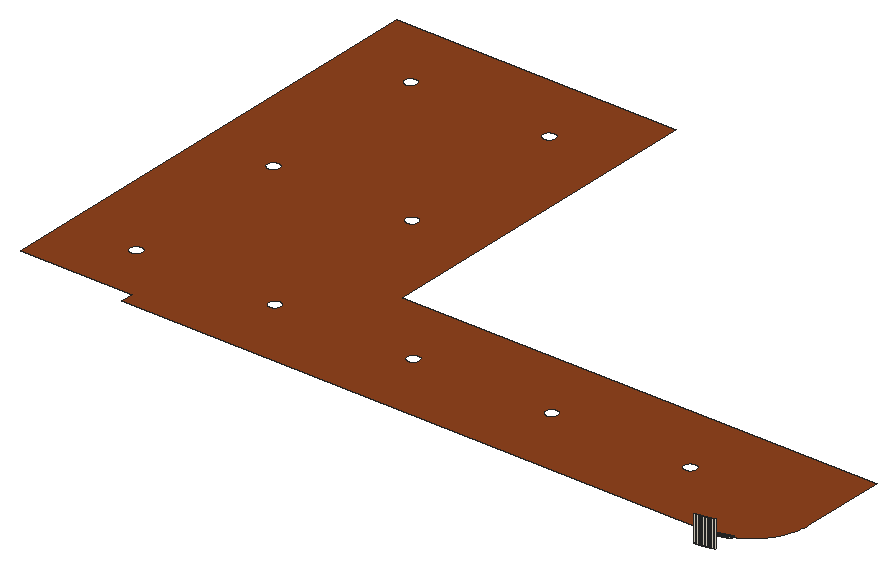
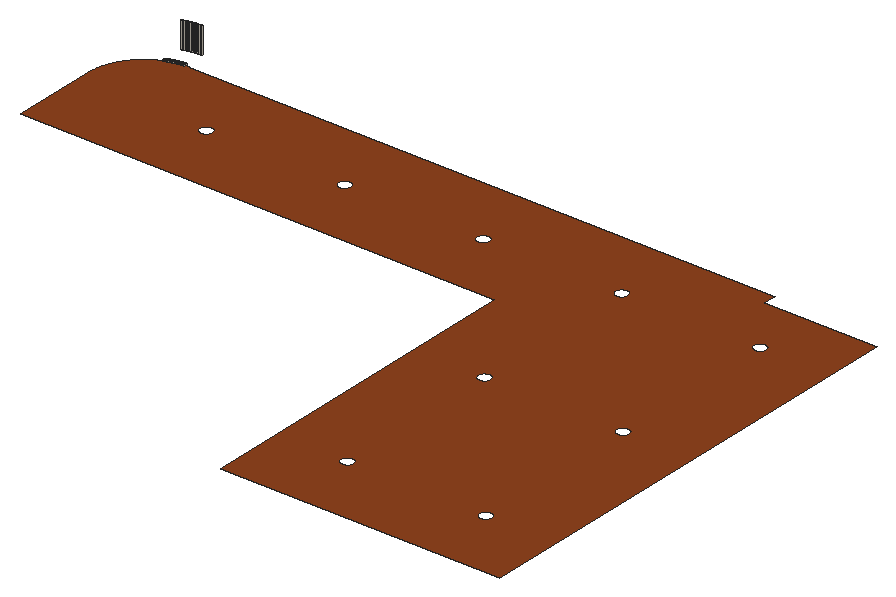
# SketchUp Ruby script. Lengths in inches.
U = 1.inch
M = Sketchup.active_model
def pt(a) = Geom::Point3d.new(a.map { |v| v * U })
def face(e, loops, mat)
  f = e.add_face(loops[0].map { |a| pt(a) })
  loops[1..].each { |l| e.add_face(l.map { |a| pt(a) }).erase! }
  f.material = f.back_material = mat if mat
  f
end
# faces: each face lists its corners as indices into pts; further lists are holes
def faces(e, pts, list, mat = nil) = list.each { |f| face(e, (f[0].is_a?(Array) ? f : [f]).map { |l| l.map { |i| pts[i] } }, mat) }
# xy, xz, yz: faces in a plane at the given z, y or x. An outline is a flat list of corners, or four numbers for a rectangle; further outlines are holes
def ring(l) = l.size == 4 ? [[l[0], l[1]], [l[2], l[1]], [l[2], l[3]], [l[0], l[3]]] : l.each_slice(2).to_a
def flat(e, list, mat, &to3) = list.each { |f| face(e, (f[0].is_a?(Array) ? f : [f]).map { |l| ring(l).map { |u, v| to3.(u, v) } }, mat) }
def xy(e, z, list, mat = nil) = flat(e, list, mat) { |x, y| [x, y, z] }
def xz(e, y, list, mat = nil) = flat(e, list, mat) { |x, z| [x, y, z] }
def yz(e, x, list, mat = nil) = flat(e, list, mat) { |y, z| [x, y, z] }
def lines(e, pts, list) = list.each { |a, b| e.add_line(pt(pts[a]), pt(pts[b])) }
# prism: a flat outline (further loops are holes) pulled along v
def prism(e, loops, v, mat = nil)
  f = face(e, loops, mat); d = Geom::Vector3d.new(v.map { |x| x * U })
  f.pushpull(f.normal.samedirection?(d) ? d.length : -d.length)
end
def box(e, o, s, mat = nil) = prism(e, [[o, [o[0] + s[0], o[1], o[2]], [o[0] + s[0], o[1] + s[1], o[2]], [o[0], o[1] + s[1], o[2]]]], [0, 0, s[2]], mat)
def at(x, y, z, deg = 0) = Geom::Transformation.translation(pt([x, y, z])) * Geom::Transformation.rotation(ORIGIN, Z_AXIS, deg.degrees)
def axes(o, x, y, z) = Geom::Transformation.new([*x, 0, *y, 0, *z, 0, *pt(o).to_a, 1])
def part(name) = M.definitions.add(name)
# library, detail: a bought-in or finely detailed component or shape, given as its bounding box
def library(name, o, s) = part(name).tap { |d| box(d.entities, o, s) }
def detail(e, o, s) = box(e.add_group.entities, o, s)
def put(e, d, t, mat = nil) = e.add_instance(d, t).tap { |i| i.material = mat if mat }
def group(e, t, mat = nil) = e.add_group.tap { |g| g.transformation = t; g.material = mat if mat }.entities
root = M.entities
M.materials.add("0027 AP L140 CRUSHED ICE").color = [241, 233, 217]
M.materials.add("[Wood Fence]").color = [142, 67, 30]
xy(root,120,[[[79,226,79,232,28,232,28,446,155,446,155,290,371,290,371,251.73,370.99,251.46,370.99,251.18,370.98,250.91,370.96,250.64,370.95,250.37,370.93,250.1,370.91,249.82,370.88,249.55,370.86,249.28,370.83,249.01,370.79,248.74,370.76,248.47,370.64,247.66,370.59,247.4,370.49,246.86,370.43,246.59,370.375,246.33,370.3125,246.0625,370.25,245.8,370.18,245.53,369.97,244.75,369.89,244.49,369.81,244.22,369.73,243.97,369.46,243.19,369.37,242.9375,369.27,242.68,369.07,242.18,368.97,241.92,368.75,241.42,368.64,241.18,368.53,240.93,368.41,240.68,368.29,240.4375,368.17,240.2,368.04,239.95,367.78,239.47,367.65,239.24,367.52,239,367.38,238.76,367.1,238.3,366.95,238.07,366.81,237.84,366.66,237.61,366.5,237.39,366.35,237.16,366.19,236.9375,366.03,236.72,365.875,236.5,365.71,236.28,365.54,236.0625,365.375,235.85,365.21,235.64,365.03,235.43,364.86,235.22,364.68,235.01,364.5,234.81,364.32,234.6,364.14,234.4,363.95,234.2,363.77,234,363.58,233.81,363.38,233.62,363.19,233.42,363,233.23,362.8,233.05,362.6,232.86,362.4,232.68,362.19,232.5,361.99,232.32,361.78,232.14,361.57,231.97,361.36,231.79,361.15,231.625,360.9375,231.46,360.72,231.29,360.5,231.125,360.28,230.97,360.0625,230.81,359.84,230.65,359.61,230.5,359.39,230.34,359.16,230.19,358.93,230.05,358.7,229.9,358.24,229.62,358,229.48,357.76,229.35,357.53,229.22,357.05,228.96,356.8,228.83,356.5625,228.71,356.32,228.59,356.07,228.47,355.82,228.36,355.58,228.25,355.08,228.03,354.82,227.93,354.32,227.73,354.0625,227.63,353.81,227.54,353.03,227.27,352.78,227.19,352.51,227.11,352.25,227.03,351.47,226.82,351.2,226.75,350.9375,226.6875,350.67,226.625,350.41,226.57,350.14,226.51,349.6,226.41,349.34,226.36,348.53,226.24,348.26,226.21,347.99,226.17,347.72,226.14,347.45,226.12,347.18,226.09,346.9,226.07,346.63,226.05,346.36,226.04,346.09,226.02,345.82,226.01,345.54,226.01,345.27,226],[311.84,255,312.16,255,312.24,255.01,312.3125,255.02,312.39,255.03,312.55,255.05,312.625,255.07,312.7,255.08,312.78,255.1,312.85,255.125,312.93,255.15,313,255.17,313.08,255.2,313.29,255.29,313.36,255.33,313.43,255.36,313.57,255.44,313.63,255.48,313.7,255.53,313.76,255.57,313.83,255.62,314.07,255.82,314.12,255.88,314.18,255.93,314.38,256.17,314.43,256.24,314.47,256.3,314.52,256.37,314.56,256.43,314.64,256.57,314.67,256.64,314.71,256.71,314.8,256.92,314.83,257,314.85,257.07,314.875,257.15,314.9,257.22,314.92,257.3,314.93,257.375,314.95,257.45,314.97,257.61,314.98,257.6875,314.99,257.76,315,257.84,315,258.16,314.99,258.24,314.98,258.3125,314.97,258.39,314.95,258.55,314.93,258.625,314.92,258.7,314.9,258.78,314.875,258.85,314.85,258.93,314.83,259,314.8,259.08,314.71,259.29,314.67,259.36,314.64,259.43,314.56,259.57,314.52,259.63,314.47,259.7,314.43,259.76,314.38,259.83,314.18,260.07,314.12,260.12,314.07,260.18,313.83,260.38,313.76,260.43,313.7,260.47,313.63,260.52,313.57,260.56,313.43,260.64,313.36,260.67,313.29,260.71,313.08,260.8,313,260.83,312.93,260.85,312.85,260.875,312.78,260.9,312.7,260.92,312.625,260.93,312.55,260.95,312.39,260.97,312.3125,260.98,312.24,260.99,312.16,261,311.84,261,311.76,260.99,311.6875,260.98,311.61,260.97,311.45,260.95,311.375,260.93,311.3,260.92,311.22,260.9,311.15,260.875,311.07,260.85,311,260.83,310.92,260.8,310.71,260.71,310.64,260.67,310.57,260.64,310.43,260.56,310.37,260.52,310.3,260.47,310.24,260.43,310.17,260.38,309.93,260.18,309.88,260.12,309.82,260.07,309.62,259.83,309.57,259.76,309.53,259.7,309.48,259.63,309.44,259.57,309.36,259.43,309.33,259.36,309.29,259.29,309.2,259.08,309.17,259,309.15,258.93,309.125,258.85,309.1,258.78,309.08,258.7,309.07,258.625,309.05,258.55,309.03,258.39,309.02,258.3125,309.01,258.24,309,258.16,309,257.84,309.01,257.76,309.02,257.6875,309.03,257.61,309.05,257.45,309.07,257.375,309.08,257.3,309.1,257.22,309.125,257.15,309.15,257.07,309.17,257,309.2,256.92,309.29,256.71,309.33,256.64,309.36,256.57,309.44,256.43,309.48,256.37,309.53,256.3,309.57,256.24,309.62,256.17,309.82,255.93,309.88,255.88,309.93,255.82,310.17,255.62,310.24,255.57,310.3,255.53,310.37,255.48,310.43,255.44,310.57,255.36,310.64,255.33,310.71,255.29,310.92,255.2,311,255.17,311.07,255.15,311.15,255.125,311.22,255.1,311.3,255.08,311.375,255.07,311.45,255.05,311.61,255.03,311.6875,255.02,311.76,255.01],[248.84,255,249.16,255,249.24,255.01,249.3125,255.02,249.39,255.03,249.55,255.05,249.625,255.07,249.7,255.08,249.78,255.1,249.85,255.125,249.93,255.15,250,255.17,250.08,255.2,250.29,255.29,250.36,255.33,250.43,255.36,250.57,255.44,250.63,255.48,250.7,255.53,250.76,255.57,250.83,255.62,251.07,255.82,251.12,255.88,251.18,255.93,251.38,256.17,251.43,256.24,251.47,256.3,251.52,256.37,251.56,256.43,251.64,256.57,251.67,256.64,251.71,256.71,251.8,256.92,251.83,257,251.85,257.07,251.875,257.15,251.9,257.22,251.92,257.3,251.93,257.375,251.95,257.45,251.97,257.61,251.98,257.6875,251.99,257.76,252,257.84,252,258.16,251.99,258.24,251.98,258.3125,251.97,258.39,251.95,258.55,251.93,258.625,251.92,258.7,251.9,258.78,251.875,258.85,251.85,258.93,251.83,259,251.8,259.08,251.71,259.29,251.67,259.36,251.64,259.43,251.56,259.57,251.52,259.63,251.47,259.7,251.43,259.76,251.38,259.83,251.18,260.07,251.12,260.12,251.07,260.18,250.83,260.38,250.76,260.43,250.7,260.47,250.63,260.52,250.57,260.56,250.43,260.64,250.36,260.67,250.29,260.71,250.08,260.8,250,260.83,249.93,260.85,249.85,260.875,249.78,260.9,249.7,260.92,249.625,260.93,249.55,260.95,249.39,260.97,249.3125,260.98,249.24,260.99,249.16,261,248.84,261,248.76,260.99,248.6875,260.98,248.61,260.97,248.45,260.95,248.375,260.93,248.3,260.92,248.22,260.9,248.15,260.875,248.07,260.85,248,260.83,247.92,260.8,247.71,260.71,247.64,260.67,247.57,260.64,247.43,260.56,247.37,260.52,247.3,260.47,247.24,260.43,247.17,260.38,246.93,260.18,246.88,260.12,246.82,260.07,246.62,259.83,246.57,259.76,246.53,259.7,246.48,259.63,246.44,259.57,246.36,259.43,246.33,259.36,246.29,259.29,246.2,259.08,246.17,259,246.15,258.93,246.125,258.85,246.1,258.78,246.08,258.7,246.07,258.625,246.05,258.55,246.03,258.39,246.02,258.3125,246.01,258.24,246,258.16,246,257.84,246.01,257.76,246.02,257.6875,246.03,257.61,246.05,257.45,246.07,257.375,246.08,257.3,246.1,257.22,246.125,257.15,246.15,257.07,246.17,257,246.2,256.92,246.29,256.71,246.33,256.64,246.36,256.57,246.44,256.43,246.48,256.37,246.53,256.3,246.57,256.24,246.62,256.17,246.82,255.93,246.88,255.88,246.93,255.82,247.17,255.62,247.24,255.57,247.3,255.53,247.37,255.48,247.43,255.44,247.57,255.36,247.64,255.33,247.71,255.29,247.92,255.2,248,255.17,248.07,255.15,248.15,255.125,248.22,255.1,248.3,255.08,248.375,255.07,248.45,255.05,248.61,255.03,248.6875,255.02,248.76,255.01],[59.84,333,60.16,333,60.24,333.01,60.3125,333.02,60.39,333.03,60.55,333.05,60.625,333.07,60.7,333.08,60.78,333.1,60.85,333.125,60.93,333.15,61,333.17,61.08,333.2,61.29,333.29,61.36,333.33,61.43,333.36,61.57,333.44,61.63,333.48,61.7,333.53,61.76,333.57,61.83,333.62,62.07,333.82,62.12,333.88,62.18,333.93,62.38,334.17,62.43,334.24,62.47,334.3,62.52,334.37,62.56,334.43,62.64,334.57,62.67,334.64,62.71,334.71,62.8,334.92,62.83,335,62.85,335.07,62.875,335.15,62.9,335.22,62.92,335.3,62.93,335.375,62.95,335.45,62.97,335.61,62.98,335.6875,62.99,335.76,63,335.84,63,336.16,62.99,336.24,62.98,336.3125,62.97,336.39,62.95,336.55,62.93,336.625,62.92,336.7,62.9,336.78,62.875,336.85,62.85,336.93,62.83,337,62.8,337.08,62.71,337.29,62.67,337.36,62.64,337.43,62.56,337.57,62.52,337.63,62.47,337.7,62.43,337.76,62.38,337.83,62.18,338.07,62.12,338.12,62.07,338.18,61.83,338.38,61.76,338.43,61.7,338.47,61.63,338.52,61.57,338.56,61.43,338.64,61.36,338.67,61.29,338.71,61.08,338.8,61,338.83,60.93,338.85,60.85,338.875,60.78,338.9,60.7,338.92,60.625,338.93,60.55,338.95,60.39,338.97,60.3125,338.98,60.24,338.99,60.16,339,59.84,339,59.76,338.99,59.6875,338.98,59.61,338.97,59.45,338.95,59.375,338.93,59.3,338.92,59.22,338.9,59.15,338.875,59.07,338.85,59,338.83,58.92,338.8,58.71,338.71,58.64,338.67,58.57,338.64,58.43,338.56,58.37,338.52,58.3,338.47,58.24,338.43,58.17,338.38,57.93,338.18,57.88,338.12,57.82,338.07,57.62,337.83,57.57,337.76,57.53,337.7,57.48,337.63,57.44,337.57,57.36,337.43,57.33,337.36,57.29,337.29,57.2,337.08,57.17,337,57.15,336.93,57.125,336.85,57.1,336.78,57.08,336.7,57.07,336.625,57.05,336.55,57.03,336.39,57.02,336.3125,57.01,336.24,57,336.16,57,335.84,57.01,335.76,57.02,335.6875,57.03,335.61,57.05,335.45,57.07,335.375,57.08,335.3,57.1,335.22,57.125,335.15,57.15,335.07,57.17,335,57.2,334.92,57.29,334.71,57.33,334.64,57.36,334.57,57.44,334.43,57.48,334.37,57.53,334.3,57.57,334.24,57.62,334.17,57.82,333.93,57.88,333.88,57.93,333.82,58.17,333.62,58.24,333.57,58.3,333.53,58.37,333.48,58.43,333.44,58.57,333.36,58.64,333.33,58.71,333.29,58.92,333.2,59,333.17,59.07,333.15,59.15,333.125,59.22,333.1,59.3,333.08,59.375,333.07,59.45,333.05,59.61,333.03,59.6875,333.02,59.76,333.01],[59.84,255,60.16,255,60.24,255.01,60.3125,255.02,60.39,255.03,60.55,255.05,60.625,255.07,60.7,255.08,60.78,255.1,60.85,255.125,60.93,255.15,61,255.17,61.08,255.2,61.29,255.29,61.36,255.33,61.43,255.36,61.57,255.44,61.63,255.48,61.7,255.53,61.76,255.57,61.83,255.62,62.07,255.82,62.12,255.88,62.18,255.93,62.38,256.17,62.43,256.24,62.47,256.3,62.52,256.37,62.56,256.43,62.64,256.57,62.67,256.64,62.71,256.71,62.8,256.92,62.83,257,62.85,257.07,62.875,257.15,62.9,257.22,62.92,257.3,62.93,257.375,62.95,257.45,62.97,257.61,62.98,257.6875,62.99,257.76,63,257.84,63,258.16,62.99,258.24,62.98,258.3125,62.97,258.39,62.95,258.55,62.93,258.625,62.92,258.7,62.9,258.78,62.875,258.85,62.85,258.93,62.83,259,62.8,259.08,62.71,259.29,62.67,259.36,62.64,259.43,62.56,259.57,62.52,259.63,62.47,259.7,62.43,259.76,62.38,259.83,62.18,260.07,62.12,260.12,62.07,260.18,61.83,260.38,61.76,260.43,61.7,260.47,61.63,260.52,61.57,260.56,61.43,260.64,61.36,260.67,61.29,260.71,61.08,260.8,61,260.83,60.93,260.85,60.85,260.875,60.78,260.9,60.7,260.92,60.625,260.93,60.55,260.95,60.39,260.97,60.3125,260.98,60.24,260.99,60.16,261,59.84,261,59.76,260.99,59.6875,260.98,59.61,260.97,59.45,260.95,59.375,260.93,59.3,260.92,59.22,260.9,59.15,260.875,59.07,260.85,59,260.83,58.92,260.8,58.71,260.71,58.64,260.67,58.57,260.64,58.43,260.56,58.37,260.52,58.3,260.47,58.24,260.43,58.17,260.38,57.93,260.18,57.88,260.12,57.82,260.07,57.62,259.83,57.57,259.76,57.53,259.7,57.48,259.63,57.44,259.57,57.36,259.43,57.33,259.36,57.29,259.29,57.2,259.08,57.17,259,57.15,258.93,57.125,258.85,57.1,258.78,57.08,258.7,57.07,258.625,57.05,258.55,57.03,258.39,57.02,258.3125,57.01,258.24,57,258.16,57,257.84,57.01,257.76,57.02,257.6875,57.03,257.61,57.05,257.45,57.07,257.375,57.08,257.3,57.1,257.22,57.125,257.15,57.15,257.07,57.17,257,57.2,256.92,57.29,256.71,57.33,256.64,57.36,256.57,57.44,256.43,57.48,256.37,57.53,256.3,57.57,256.24,57.62,256.17,57.82,255.93,57.88,255.88,57.93,255.82,58.17,255.62,58.24,255.57,58.3,255.53,58.37,255.48,58.43,255.44,58.57,255.36,58.64,255.33,58.71,255.29,58.92,255.2,59,255.17,59.07,255.15,59.15,255.125,59.22,255.1,59.3,255.08,59.375,255.07,59.45,255.05,59.61,255.03,59.6875,255.02,59.76,255.01],[122.84,411,123.16,411,123.24,411.01,123.3125,411.02,123.39,411.03,123.55,411.05,123.625,411.07,123.7,411.08,123.78,411.1,123.85,411.125,123.93,411.15,124,411.17,124.08,411.2,124.29,411.29,124.36,411.33,124.43,411.36,124.57,411.44,124.63,411.48,124.7,411.53,124.76,411.57,124.83,411.62,125.07,411.82,125.12,411.88,125.18,411.93,125.38,412.17,125.43,412.24,125.47,412.3,125.52,412.37,125.56,412.43,125.64,412.57,125.67,412.64,125.71,412.71,125.8,412.92,125.83,413,125.85,413.07,125.875,413.15,125.9,413.22,125.92,413.3,125.93,413.375,125.95,413.45,125.97,413.61,125.98,413.6875,125.99,413.76,126,413.84,126,414.16,125.99,414.24,125.98,414.3125,125.97,414.39,125.95,414.55,125.93,414.625,125.92,414.7,125.9,414.78,125.875,414.85,125.85,414.93,125.83,415,125.8,415.08,125.71,415.29,125.67,415.36,125.64,415.43,125.56,415.57,125.52,415.63,125.47,415.7,125.43,415.76,125.38,415.83,125.18,416.07,125.12,416.12,125.07,416.18,124.83,416.38,124.76,416.43,124.7,416.47,124.63,416.52,124.57,416.56,124.43,416.64,124.36,416.67,124.29,416.71,124.08,416.8,124,416.83,123.93,416.85,123.85,416.875,123.78,416.9,123.7,416.92,123.625,416.93,123.55,416.95,123.39,416.97,123.3125,416.98,123.24,416.99,123.16,417,122.84,417,122.76,416.99,122.6875,416.98,122.61,416.97,122.45,416.95,122.375,416.93,122.3,416.92,122.22,416.9,122.15,416.875,122.07,416.85,122,416.83,121.92,416.8,121.71,416.71,121.64,416.67,121.57,416.64,121.43,416.56,121.37,416.52,121.3,416.47,121.24,416.43,121.17,416.38,120.93,416.18,120.88,416.12,120.82,416.07,120.62,415.83,120.57,415.76,120.53,415.7,120.48,415.63,120.44,415.57,120.36,415.43,120.33,415.36,120.29,415.29,120.2,415.08,120.17,415,120.15,414.93,120.125,414.85,120.1,414.78,120.08,414.7,120.07,414.625,120.05,414.55,120.03,414.39,120.02,414.3125,120.01,414.24,120,414.16,120,413.84,120.01,413.76,120.02,413.6875,120.03,413.61,120.05,413.45,120.07,413.375,120.08,413.3,120.1,413.22,120.125,413.15,120.15,413.07,120.17,413,120.2,412.92,120.29,412.71,120.33,412.64,120.36,412.57,120.44,412.43,120.48,412.37,120.53,412.3,120.57,412.24,120.62,412.17,120.82,411.93,120.88,411.88,120.93,411.82,121.17,411.62,121.24,411.57,121.3,411.53,121.37,411.48,121.43,411.44,121.57,411.36,121.64,411.33,121.71,411.29,121.92,411.2,122,411.17,122.07,411.15,122.15,411.125,122.22,411.1,122.3,411.08,122.375,411.07,122.45,411.05,122.61,411.03,122.6875,411.02,122.76,411.01],[122.84,333,123.16,333,123.24,333.01,123.3125,333.02,123.39,333.03,123.55,333.05,123.625,333.07,123.7,333.08,123.78,333.1,123.85,333.125,123.93,333.15,124,333.17,124.08,333.2,124.29,333.29,124.36,333.33,124.43,333.36,124.57,333.44,124.63,333.48,124.7,333.53,124.76,333.57,124.83,333.62,125.07,333.82,125.12,333.88,125.18,333.93,125.38,334.17,125.43,334.24,125.47,334.3,125.52,334.37,125.56,334.43,125.64,334.57,125.67,334.64,125.71,334.71,125.8,334.92,125.83,335,125.85,335.07,125.875,335.15,125.9,335.22,125.92,335.3,125.93,335.375,125.95,335.45,125.97,335.61,125.98,335.6875,125.99,335.76,126,335.84,126,336.16,125.99,336.24,125.98,336.3125,125.97,336.39,125.95,336.55,125.93,336.625,125.92,336.7,125.9,336.78,125.875,336.85,125.85,336.93,125.83,337,125.8,337.08,125.71,337.29,125.67,337.36,125.64,337.43,125.56,337.57,125.52,337.63,125.47,337.7,125.43,337.76,125.38,337.83,125.18,338.07,125.12,338.12,125.07,338.18,124.83,338.38,124.76,338.43,124.7,338.47,124.63,338.52,124.57,338.56,124.43,338.64,124.36,338.67,124.29,338.71,124.08,338.8,124,338.83,123.93,338.85,123.85,338.875,123.78,338.9,123.7,338.92,123.625,338.93,123.55,338.95,123.39,338.97,123.3125,338.98,123.24,338.99,123.16,339,122.84,339,122.76,338.99,122.6875,338.98,122.61,338.97,122.45,338.95,122.375,338.93,122.3,338.92,122.22,338.9,122.15,338.875,122.07,338.85,122,338.83,121.92,338.8,121.71,338.71,121.64,338.67,121.57,338.64,121.43,338.56,121.37,338.52,121.3,338.47,121.24,338.43,121.17,338.38,120.93,338.18,120.88,338.12,120.82,338.07,120.62,337.83,120.57,337.76,120.53,337.7,120.48,337.63,120.44,337.57,120.36,337.43,120.33,337.36,120.29,337.29,120.2,337.08,120.17,337,120.15,336.93,120.125,336.85,120.1,336.78,120.08,336.7,120.07,336.625,120.05,336.55,120.03,336.39,120.02,336.3125,120.01,336.24,120,336.16,120,335.84,120.01,335.76,120.02,335.6875,120.03,335.61,120.05,335.45,120.07,335.375,120.08,335.3,120.1,335.22,120.125,335.15,120.15,335.07,120.17,335,120.2,334.92,120.29,334.71,120.33,334.64,120.36,334.57,120.44,334.43,120.48,334.37,120.53,334.3,120.57,334.24,120.62,334.17,120.82,333.93,120.88,333.88,120.93,333.82,121.17,333.62,121.24,333.57,121.3,333.53,121.37,333.48,121.43,333.44,121.57,333.36,121.64,333.33,121.71,333.29,121.92,333.2,122,333.17,122.07,333.15,122.15,333.125,122.22,333.1,122.3,333.08,122.375,333.07,122.45,333.05,122.61,333.03,122.6875,333.02,122.76,333.01],[122.84,255,123.16,255,123.24,255.01,123.3125,255.02,123.39,255.03,123.55,255.05,123.625,255.07,123.7,255.08,123.78,255.1,123.85,255.125,123.93,255.15,124,255.17,124.08,255.2,124.29,255.29,124.36,255.33,124.43,255.36,124.57,255.44,124.63,255.48,124.7,255.53,124.76,255.57,124.83,255.62,125.07,255.82,125.12,255.88,125.18,255.93,125.38,256.17,125.43,256.24,125.47,256.3,125.52,256.37,125.56,256.43,125.64,256.57,125.67,256.64,125.71,256.71,125.8,256.92,125.83,257,125.85,257.07,125.875,257.15,125.9,257.22,125.92,257.3,125.93,257.375,125.95,257.45,125.97,257.61,125.98,257.6875,125.99,257.76,126,257.84,126,258.16,125.99,258.24,125.98,258.3125,125.97,258.39,125.95,258.55,125.93,258.625,125.92,258.7,125.9,258.78,125.875,258.85,125.85,258.93,125.83,259,125.8,259.08,125.71,259.29,125.67,259.36,125.64,259.43,125.56,259.57,125.52,259.63,125.47,259.7,125.43,259.76,125.38,259.83,125.18,260.07,125.12,260.12,125.07,260.18,124.83,260.38,124.76,260.43,124.7,260.47,124.63,260.52,124.57,260.56,124.43,260.64,124.36,260.67,124.29,260.71,124.08,260.8,124,260.83,123.93,260.85,123.85,260.875,123.78,260.9,123.7,260.92,123.625,260.93,123.55,260.95,123.39,260.97,123.3125,260.98,123.24,260.99,123.16,261,122.84,261,122.76,260.99,122.6875,260.98,122.61,260.97,122.45,260.95,122.375,260.93,122.3,260.92,122.22,260.9,122.15,260.875,122.07,260.85,122,260.83,121.92,260.8,121.71,260.71,121.64,260.67,121.57,260.64,121.43,260.56,121.37,260.52,121.3,260.47,121.24,260.43,121.17,260.38,120.93,260.18,120.88,260.12,120.82,260.07,120.62,259.83,120.57,259.76,120.53,259.7,120.48,259.63,120.44,259.57,120.36,259.43,120.33,259.36,120.29,259.29,120.2,259.08,120.17,259,120.15,258.93,120.125,258.85,120.1,258.78,120.08,258.7,120.07,258.625,120.05,258.55,120.03,258.39,120.02,258.3125,120.01,258.24,120,258.16,120,257.84,120.01,257.76,120.02,257.6875,120.03,257.61,120.05,257.45,120.07,257.375,120.08,257.3,120.1,257.22,120.125,257.15,120.15,257.07,120.17,257,120.2,256.92,120.29,256.71,120.33,256.64,120.36,256.57,120.44,256.43,120.48,256.37,120.53,256.3,120.57,256.24,120.62,256.17,120.82,255.93,120.88,255.88,120.93,255.82,121.17,255.62,121.24,255.57,121.3,255.53,121.37,255.48,121.43,255.44,121.57,255.36,121.64,255.33,121.71,255.29,121.92,255.2,122,255.17,122.07,255.15,122.15,255.125,122.22,255.1,122.3,255.08,122.375,255.07,122.45,255.05,122.61,255.03,122.6875,255.02,122.76,255.01],[185.84,255,186.16,255,186.24,255.01,186.3125,255.02,186.39,255.03,186.55,255.05,186.625,255.07,186.7,255.08,186.78,255.1,186.85,255.125,186.93,255.15,187,255.17,187.08,255.2,187.29,255.29,187.36,255.33,187.43,255.36,187.57,255.44,187.63,255.48,187.7,255.53,187.76,255.57,187.83,255.62,188.07,255.82,188.12,255.88,188.18,255.93,188.38,256.17,188.43,256.24,188.47,256.3,188.52,256.37,188.56,256.43,188.64,256.57,188.67,256.64,188.71,256.71,188.8,256.92,188.83,257,188.85,257.07,188.875,257.15,188.9,257.22,188.92,257.3,188.93,257.375,188.95,257.45,188.97,257.61,188.98,257.6875,188.99,257.76,189,257.84,189,258.16,188.99,258.24,188.98,258.3125,188.97,258.39,188.95,258.55,188.93,258.625,188.92,258.7,188.9,258.78,188.875,258.85,188.85,258.93,188.83,259,188.8,259.08,188.71,259.29,188.67,259.36,188.64,259.43,188.56,259.57,188.52,259.63,188.47,259.7,188.43,259.76,188.38,259.83,188.18,260.07,188.12,260.12,188.07,260.18,187.83,260.38,187.76,260.43,187.7,260.47,187.63,260.52,187.57,260.56,187.43,260.64,187.36,260.67,187.29,260.71,187.08,260.8,187,260.83,186.93,260.85,186.85,260.875,186.78,260.9,186.7,260.92,186.625,260.93,186.55,260.95,186.39,260.97,186.3125,260.98,186.24,260.99,186.16,261,185.84,261,185.76,260.99,185.6875,260.98,185.61,260.97,185.45,260.95,185.375,260.93,185.3,260.92,185.22,260.9,185.15,260.875,185.07,260.85,185,260.83,184.92,260.8,184.71,260.71,184.64,260.67,184.57,260.64,184.43,260.56,184.37,260.52,184.3,260.47,184.24,260.43,184.17,260.38,183.93,260.18,183.88,260.12,183.82,260.07,183.62,259.83,183.57,259.76,183.53,259.7,183.48,259.63,183.44,259.57,183.36,259.43,183.33,259.36,183.29,259.29,183.2,259.08,183.17,259,183.15,258.93,183.125,258.85,183.1,258.78,183.08,258.7,183.07,258.625,183.05,258.55,183.03,258.39,183.02,258.3125,183.01,258.24,183,258.16,183,257.84,183.01,257.76,183.02,257.6875,183.03,257.61,183.05,257.45,183.07,257.375,183.08,257.3,183.1,257.22,183.125,257.15,183.15,257.07,183.17,257,183.2,256.92,183.29,256.71,183.33,256.64,183.36,256.57,183.44,256.43,183.48,256.37,183.53,256.3,183.57,256.24,183.62,256.17,183.82,255.93,183.88,255.88,183.93,255.82,184.17,255.62,184.24,255.57,184.3,255.53,184.37,255.48,184.43,255.44,184.57,255.36,184.64,255.33,184.71,255.29,184.92,255.2,185,255.17,185.07,255.15,185.15,255.125,185.22,255.1,185.3,255.08,185.375,255.07,185.45,255.05,185.61,255.03,185.6875,255.02,185.76,255.01],[59.84,411,60.16,411,60.24,411.01,60.3125,411.02,60.39,411.03,60.55,411.05,60.625,411.07,60.7,411.08,60.78,411.1,60.85,411.125,60.93,411.15,61,411.17,61.08,411.2,61.29,411.29,61.36,411.33,61.43,411.36,61.57,411.44,61.63,411.48,61.7,411.53,61.76,411.57,61.83,411.62,62.07,411.82,62.12,411.88,62.18,411.93,62.38,412.17,62.43,412.24,62.47,412.3,62.52,412.37,62.56,412.43,62.64,412.57,62.67,412.64,62.71,412.71,62.8,412.92,62.83,413,62.85,413.07,62.875,413.15,62.9,413.22,62.92,413.3,62.93,413.375,62.95,413.45,62.97,413.61,62.98,413.6875,62.99,413.76,63,413.84,63,414.16,62.99,414.24,62.98,414.3125,62.97,414.39,62.95,414.55,62.93,414.625,62.92,414.7,62.9,414.78,62.875,414.85,62.85,414.93,62.83,415,62.8,415.08,62.71,415.29,62.67,415.36,62.64,415.43,62.56,415.57,62.52,415.63,62.47,415.7,62.43,415.76,62.38,415.83,62.18,416.07,62.12,416.12,62.07,416.18,61.83,416.38,61.76,416.43,61.7,416.47,61.63,416.52,61.57,416.56,61.43,416.64,61.36,416.67,61.29,416.71,61.08,416.8,61,416.83,60.93,416.85,60.85,416.875,60.78,416.9,60.7,416.92,60.625,416.93,60.55,416.95,60.39,416.97,60.3125,416.98,60.24,416.99,60.16,417,59.84,417,59.76,416.99,59.6875,416.98,59.61,416.97,59.45,416.95,59.375,416.93,59.3,416.92,59.22,416.9,59.15,416.875,59.07,416.85,59,416.83,58.92,416.8,58.71,416.71,58.64,416.67,58.57,416.64,58.43,416.56,58.37,416.52,58.3,416.47,58.24,416.43,58.17,416.38,57.93,416.18,57.88,416.12,57.82,416.07,57.62,415.83,57.57,415.76,57.53,415.7,57.48,415.63,57.44,415.57,57.36,415.43,57.33,415.36,57.29,415.29,57.2,415.08,57.17,415,57.15,414.93,57.125,414.85,57.1,414.78,57.08,414.7,57.07,414.625,57.05,414.55,57.03,414.39,57.02,414.3125,57.01,414.24,57,414.16,57,413.84,57.01,413.76,57.02,413.6875,57.03,413.61,57.05,413.45,57.07,413.375,57.08,413.3,57.1,413.22,57.125,413.15,57.15,413.07,57.17,413,57.2,412.92,57.29,412.71,57.33,412.64,57.36,412.57,57.44,412.43,57.48,412.37,57.53,412.3,57.57,412.24,57.62,412.17,57.82,411.93,57.88,411.88,57.93,411.82,58.17,411.62,58.24,411.57,58.3,411.53,58.37,411.48,58.43,411.44,58.57,411.36,58.64,411.33,58.71,411.29,58.92,411.2,59,411.17,59.07,411.15,59.15,411.125,59.22,411.1,59.3,411.08,59.375,411.07,59.45,411.05,59.61,411.03,59.6875,411.02,59.76,411.01]]],"[Wood Fence]")
p = [[347.64,216.1,132],[347.26,216.07,132],[347.26,216.07,120],[347.64,216.1,120],[348.01,216.125,132],[348.01,216.125,120],
  [348.39,216.16,132],[348.39,216.16,120],[348.76,216.2,132],[348.76,216.2,120],[349.14,216.24,132],[349.14,216.24,120],
  [349.51,216.28,132],[349.51,216.28,120],[349.89,216.33,132],[349.89,216.33,120],[350.26,216.39,132],[350.26,216.39,120],
  [350.63,216.44,132],[350.63,216.44,120],[351,216.5,132],[351,216.5,120],[351.375,216.57,132],[351.375,216.57,120],
  [351.75,216.64,132],[351.75,216.64,120],[352.12,216.71,132],[352.12,216.71,120],[352.48,216.79,132],[352.48,216.79,120],
  [352.85,216.87,132],[352.85,216.87,120],[353.22,216.95,132],[353.22,216.95,120],[353.59,217.04,132],[353.59,217.04,120],
  [353.95,217.13,132],[353.95,217.13,120],[354.32,217.23,132],[354.32,217.23,120],[354.68,217.33,132],[354.68,217.33,120],
  [355.04,217.43,132],[355.04,217.43,120],[355.41,217.54,132],[355.41,217.54,120],[355.77,217.65,132],[355.77,217.65,120],
  [347.54,225.12,120],[347.26,225.09,120],[347.26,225.09,120.5],[347.54,225.12,120.5],[347.82,225.15,120],[347.82,225.15,120.5],
  [348.1,225.18,120],[348.1,225.18,120.5],[348.38,225.21,120],[348.38,225.21,120.5],[348.66,225.25,120],[348.66,225.25,120.5],
  [348.94,225.29,120],[348.94,225.29,120.5],[349.22,225.33,120],[349.22,225.33,120.5],[349.5,225.38,120],[349.5,225.38,120.5],
  [349.78,225.43,120],[349.78,225.43,120.5],[350.06,225.48,120],[350.06,225.48,120.5],[350.34,225.53,120],[350.34,225.53,120.5],
  [350.61,225.59,120],[350.61,225.59,120.5],[350.89,225.65,120],[350.89,225.65,120.5],[351.17,225.71,120],[351.17,225.71,120.5],
  [351.44,225.78,120],[351.44,225.78,120.5],[351.71,225.85,120],[351.71,225.85,120.5],[351.99,225.92,120],[351.99,225.92,120.5],
  [352.26,225.99,120],[352.26,225.99,120.5],[352.53,226.07,120],[352.53,226.07,120.5],[347.45,226.12,120],[347.72,226.14,120],
  [347.72,226.14,120.5],[347.45,226.12,120.5],[347.99,226.17,120],[347.99,226.17,120.5],[352.8,226.15,120],[352.8,226.15,120.5],
  [348.26,226.21,120],[348.26,226.21,120.5],[348.53,226.24,120],[348.53,226.24,120.5],[348.8,226.28,120],[348.8,226.28,120.5],
  [353.07,226.24,120],[353.07,226.24,120.5],[353.34,226.32,120],[353.34,226.32,120.5],[349.07,226.32,120],[349.07,226.32,120.5],
  [349.34,226.36,120],[349.34,226.36,120.5],[353.61,226.41,120],[353.61,226.41,120.5],[349.6,226.41,120],[349.6,226.41,120.5],
  [349.87,226.46,120],[349.87,226.46,120.5],[353.88,226.5,120],[353.88,226.5,120.5],[350.14,226.51,120],[350.14,226.51,120.5],
  [350.41,226.57,120],[350.41,226.57,120.5],[354.15,226.6,120],[354.15,226.6,120.5],[350.67,226.625,120],[350.67,226.625,120.5],
  [350.9375,226.6875,120],[350.9375,226.6875,120.5],[354.41,226.69,120],[354.41,226.69,120.5],[351.2,226.75,120],[351.2,226.75,120.5],
  [354.68,226.79,120],[354.68,226.79,120.5],[351.47,226.82,120],[351.47,226.82,120.5],[351.73,226.89,120],[351.73,226.89,120.5],
  [354.9375,226.9,120],[354.9375,226.9,120.5],[351.99,226.96,120],[351.99,226.96,120.5],[355.2,227,120],[355.2,227,120.5],
  [352.25,227.03,120],[352.25,227.03,120.5],[352.51,227.11,120],[352.51,227.11,120.5],[355.46,227.11,120],[355.46,227.11,120.5],
  [352.78,227.19,120],[352.78,227.19,120.5],[355.72,227.22,120],[355.72,227.22,120.5],[353.03,227.27,120],[353.03,227.27,120.5],
  [353.29,227.36,120],[353.29,227.36,120.5],[353.55,227.45,120],[353.55,227.45,120.5],[353.81,227.54,120],[353.81,227.54,120.5],
  [354.0625,227.63,120],[354.0625,227.63,120.5],[354.32,227.73,120],[354.32,227.73,120.5],[354.57,227.83,120],[354.57,227.83,120.5],
  [354.82,227.93,120],[354.82,227.93,120.5],[355.08,228.03,120],[355.08,228.03,120.5],[355.33,228.14,120],[355.33,228.14,120.5],
  [355.58,228.25,120],[355.58,228.25,120.5]]
faces(root,p,[[0,1,2,3],[4,0,3,5],[6,4,5,7],[8,6,7,9],[10,8,9,11],[12,10,11,13],[14,12,13,15],[16,14,15,17],
  [18,16,17,19],[20,18,19,21],[22,20,21,23],[24,22,23,25],[26,24,25,27],[28,26,27,29],[30,28,29,31],[32,30,31,33],
  [34,32,33,35],[36,34,35,37],[38,36,37,39],[40,38,39,41],[42,40,41,43],[44,42,43,45],[46,44,45,47],[48,49,50,51],
  [52,48,51,53],[54,52,53,55],[56,54,55,57],[58,56,57,59],[60,58,59,61],[62,60,61,63],[64,62,63,65],[66,64,65,67],
  [68,66,67,69],[70,68,69,71],[72,70,71,73],[74,72,73,75],[76,74,75,77],[78,76,77,79],[80,78,79,81],[82,80,81,83],
  [84,82,83,85],[86,84,85,87],[88,89,90,91],[89,92,93,90],[94,86,87,95],[92,96,97,93],[96,98,99,97],[98,100,101,99],
  [102,94,95,103],[104,102,103,105],[100,106,107,101],[106,108,109,107],[110,104,105,111],[108,112,113,109],[112,114,115,113],[116,110,111,117],
  [114,118,119,115],[118,120,121,119],[122,116,117,123],[120,124,125,121],[124,126,127,125],[128,122,123,129],[126,130,131,127],[132,128,129,133],
  [130,134,135,131],[134,136,137,135],[138,132,133,139],[136,140,141,137],[142,138,139,143],[140,144,145,141],[144,146,147,145],[148,142,143,149],
  [146,150,151,147],[152,148,149,153],[150,154,155,151],[154,156,157,155],[156,158,159,157],[158,160,161,159],[160,162,163,161],[162,164,165,163],
  [164,166,167,165],[166,168,169,167],[168,170,171,169],[170,172,173,171],[172,174,175,173]],"0027 AP L140 CRUSHED ICE")
